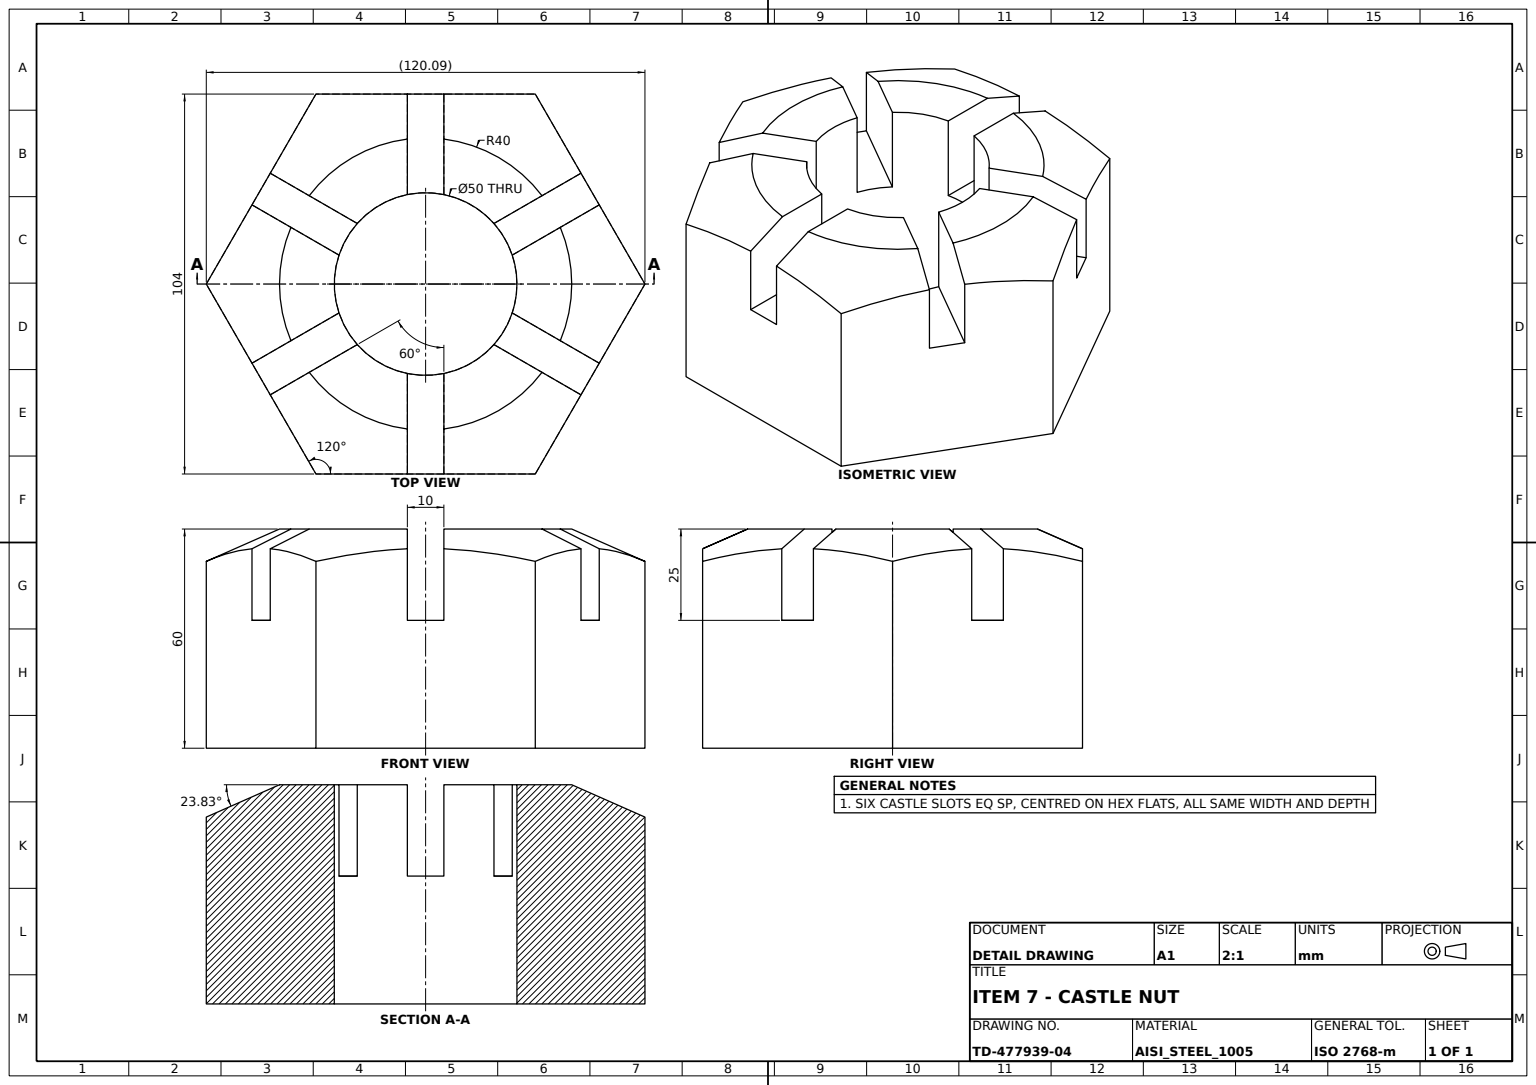
ISO-10303-21;
HEADER;
FILE_DESCRIPTION((''),'2;1');
FILE_NAME('','',(''),(''),'','','');
FILE_SCHEMA(('AUTOMOTIVE_DESIGN'));
ENDSEC;
DATA;
#1=APPLICATION_CONTEXT('');
#2=PRODUCT_CONTEXT('',#1,'mechanical');
#3=PRODUCT('','','',(#2));
#4=PRODUCT_DEFINITION_FORMATION('','',#3);
#5=PRODUCT_DEFINITION_CONTEXT('',#1,'design');
#6=PRODUCT_DEFINITION('','',#4,#5);
#7=PRODUCT_DEFINITION_SHAPE('','',#6);
#8=(LENGTH_UNIT()NAMED_UNIT(*)SI_UNIT(.MILLI.,.METRE.));
#9=(NAMED_UNIT(*)PLANE_ANGLE_UNIT()SI_UNIT($,.RADIAN.));
#10=(NAMED_UNIT(*)SI_UNIT($,.STERADIAN.)SOLID_ANGLE_UNIT());
#11=UNCERTAINTY_MEASURE_WITH_UNIT(LENGTH_MEASURE(0.005),#8,'distance_accuracy_value','');
#12=(GEOMETRIC_REPRESENTATION_CONTEXT(3)GLOBAL_UNCERTAINTY_ASSIGNED_CONTEXT((#11))GLOBAL_UNIT_ASSIGNED_CONTEXT((#8,#9,#10))REPRESENTATION_CONTEXT('',''));
#13=CARTESIAN_POINT('',(-47.533321,21.669873,54.594675));
#14=VERTEX_POINT('',#13);
#15=CARTESIAN_POINT('',(-36.869318,15.513008,60.));
#16=VERTEX_POINT('',#15);
#17=CARTESIAN_POINT('',(-47.533323,21.669874,54.594679));
#18=CARTESIAN_POINT('',(-43.979469,19.618056,56.398596));
#19=CARTESIAN_POINT('',(-40.425051,17.565911,58.201027));
#20=B_SPLINE_CURVE_WITH_KNOTS('',3,(#17,#18,#19,#15),.UNSPECIFIED.,.F.,.F.,(4,4),(0.00000025,0.013448131),.UNSPECIFIED.);
#21=EDGE_CURVE('',#14,#16,#20,.T.);
#22=ORIENTED_EDGE('',*,*,#21,.F.);
#23=CARTESIAN_POINT('',(-60.044428,0.,51.148036));
#24=VERTEX_POINT('',#23);
#25=CARTESIAN_POINT('',(-55.892067,7.1921,52.98179));
#26=CARTESIAN_POINT('',(-51.724583,14.410395,54.240365));
#27=CARTESIAN_POINT('',(-47.533321,21.669873,54.59468));
#28=B_SPLINE_CURVE_WITH_KNOTS('',3,(#23,#25,#26,#27),.UNSPECIFIED.,.F.,.F.,(4,4),(0.000000233,0.025168923),.UNSPECIFIED.);
#29=EDGE_CURVE('',#24,#14,#28,.T.);
#30=ORIENTED_EDGE('',*,*,#29,.F.);
#31=CARTESIAN_POINT('',(-47.533321,-21.669873,54.594675));
#32=VERTEX_POINT('',#31);
#33=CARTESIAN_POINT('',(-47.533321,-21.669873,54.59468));
#34=CARTESIAN_POINT('',(-49.619911,-18.055793,54.418287));
#35=CARTESIAN_POINT('',(-53.818812,-10.783084,53.616325));
#36=CARTESIAN_POINT('',(-57.97964,-3.576317,52.059882));
#37=B_SPLINE_CURVE_WITH_KNOTS('',3,(#33,#34,#35,#36,#23),.UNSPECIFIED.,.F.,.F.,(4,1,4),(0.035155124,0.047629599,0.060104073),.UNSPECIFIED.);
#38=EDGE_CURVE('',#32,#24,#37,.T.);
#39=ORIENTED_EDGE('',*,*,#38,.F.);
#40=CARTESIAN_POINT('',(-36.869318,-15.513008,60.));
#41=VERTEX_POINT('',#40);
#42=CARTESIAN_POINT('',(-40.425051,-17.565911,58.201027));
#43=CARTESIAN_POINT('',(-43.979469,-19.618056,56.398596));
#44=CARTESIAN_POINT('',(-47.533323,-21.669874,54.594679));
#45=B_SPLINE_CURVE_WITH_KNOTS('',3,(#40,#42,#43,#44),.UNSPECIFIED.,.F.,.F.,(4,4),(0.000000498,0.013448379),.UNSPECIFIED.);
#46=EDGE_CURVE('',#41,#32,#45,.T.);
#47=ORIENTED_EDGE('',*,*,#46,.F.);
#48=CARTESIAN_POINT('',(0.,0.,60.));
#49=DIRECTION('',(0.,0.,-1.));
#50=DIRECTION('',(-1.,0.,0.));
#51=AXIS2_PLACEMENT_3D('',#48,#49,#50);
#52=CIRCLE('',#51,40.);
#53=EDGE_CURVE('',#41,#16,#52,.T.);
#54=ORIENTED_EDGE('',*,*,#53,.T.);
#55=EDGE_LOOP('',(#22,#30,#39,#47,#54));
#56=FACE_BOUND('',#55,.T.);
#57=CONICAL_SURFACE('',#51,40.,1.154935364);
#58=ADVANCED_FACE('',(#56),#57,.T.);
#59=CARTESIAN_POINT('',(-5.,-52.,54.59468));
#60=VERTEX_POINT('',#59);
#61=CARTESIAN_POINT('',(-5.,-39.68627,60.));
#62=VERTEX_POINT('',#61);
#63=CARTESIAN_POINT('',(-5.,-47.89636,56.398598));
#64=CARTESIAN_POINT('',(-5.,-43.792065,58.201031));
#65=B_SPLINE_CURVE_WITH_KNOTS('',3,(#59,#63,#64,#61),.UNSPECIFIED.,.F.,.F.,(4,4),(0.047300032,0.060747922),.UNSPECIFIED.);
#66=EDGE_CURVE('',#60,#62,#65,.T.);
#67=ORIENTED_EDGE('',*,*,#66,.T.);
#68=CARTESIAN_POINT('',(-31.869318,-24.173262,60.));
#69=VERTEX_POINT('',#68);
#70=EDGE_CURVE('',#62,#69,#52,.T.);
#71=ORIENTED_EDGE('',*,*,#70,.T.);
#72=CARTESIAN_POINT('',(-42.533321,-30.330127,54.594675));
#73=VERTEX_POINT('',#72);
#74=CARTESIAN_POINT('',(-42.533323,-30.330128,54.594679));
#75=CARTESIAN_POINT('',(-38.979469,-28.27831,56.398596));
#76=CARTESIAN_POINT('',(-35.425051,-26.226165,58.201027));
#77=B_SPLINE_CURVE_WITH_KNOTS('',3,(#74,#75,#76,#68),.UNSPECIFIED.,.F.,.F.,(4,4),(0.00000025,0.013448131),.UNSPECIFIED.);
#78=EDGE_CURVE('',#73,#69,#77,.T.);
#79=ORIENTED_EDGE('',*,*,#78,.F.);
#80=CARTESIAN_POINT('',(-30.022214,-52.,51.148036));
#81=VERTEX_POINT('',#80);
#82=CARTESIAN_POINT('',(-34.174575,-44.8079,52.98179));
#83=CARTESIAN_POINT('',(-38.342059,-37.589605,54.240365));
#84=CARTESIAN_POINT('',(-42.533321,-30.330127,54.59468));
#85=B_SPLINE_CURVE_WITH_KNOTS('',3,(#80,#82,#83,#84),.UNSPECIFIED.,.F.,.F.,(4,4),(0.000000233,0.025168923),.UNSPECIFIED.);
#86=EDGE_CURVE('',#81,#73,#85,.T.);
#87=ORIENTED_EDGE('',*,*,#86,.F.);
#88=CARTESIAN_POINT('',(-25.899769,-52.,52.058307));
#89=CARTESIAN_POINT('',(-17.542965,-52.,53.620138));
#90=CARTESIAN_POINT('',(-9.18181,-52.,54.417922));
#91=B_SPLINE_CURVE_WITH_KNOTS('',3,(#80,#88,#89,#90,#59),.UNSPECIFIED.,.F.,.F.,(4,1,4),(0.051261487,0.063895866,0.076530245),.UNSPECIFIED.);
#92=EDGE_CURVE('',#60,#81,#91,.F.);
#93=ORIENTED_EDGE('',*,*,#92,.F.);
#94=EDGE_LOOP('',(#67,#71,#79,#87,#93));
#95=FACE_BOUND('',#94,.T.);
#96=ADVANCED_FACE('',(#95),#57,.T.);
#97=CARTESIAN_POINT('',(-42.533321,30.330127,54.594675));
#98=VERTEX_POINT('',#97);
#99=CARTESIAN_POINT('',(-30.022214,52.,51.148036));
#100=VERTEX_POINT('',#99);
#101=CARTESIAN_POINT('',(-42.533321,30.330127,54.59468));
#102=CARTESIAN_POINT('',(-40.446731,33.944207,54.418287));
#103=CARTESIAN_POINT('',(-36.24783,41.216916,53.616325));
#104=CARTESIAN_POINT('',(-32.087002,48.423683,52.059882));
#105=B_SPLINE_CURVE_WITH_KNOTS('',3,(#101,#102,#103,#104,#99),.UNSPECIFIED.,.F.,.F.,(4,1,4),(0.035155124,0.047629599,0.060104073),.UNSPECIFIED.);
#106=EDGE_CURVE('',#98,#100,#105,.T.);
#107=ORIENTED_EDGE('',*,*,#106,.F.);
#108=CARTESIAN_POINT('',(-31.869318,24.173262,60.));
#109=VERTEX_POINT('',#108);
#110=CARTESIAN_POINT('',(-35.425051,26.226165,58.201027));
#111=CARTESIAN_POINT('',(-38.979469,28.27831,56.398596));
#112=CARTESIAN_POINT('',(-42.533323,30.330128,54.594679));
#113=B_SPLINE_CURVE_WITH_KNOTS('',3,(#108,#110,#111,#112),.UNSPECIFIED.,.F.,.F.,(4,4),(0.000000498,0.013448379),.UNSPECIFIED.);
#114=EDGE_CURVE('',#109,#98,#113,.T.);
#115=ORIENTED_EDGE('',*,*,#114,.F.);
#116=CARTESIAN_POINT('',(-5.,39.68627,60.));
#117=VERTEX_POINT('',#116);
#118=EDGE_CURVE('',#109,#117,#52,.T.);
#119=ORIENTED_EDGE('',*,*,#118,.T.);
#120=CARTESIAN_POINT('',(-5.,52.,54.59468));
#121=VERTEX_POINT('',#120);
#122=CARTESIAN_POINT('',(-5.,43.792075,58.201027));
#123=CARTESIAN_POINT('',(-5.,47.896365,56.398596));
#124=B_SPLINE_CURVE_WITH_KNOTS('',3,(#116,#122,#123,#120),.UNSPECIFIED.,.F.,.F.,(4,4),(0.029122538,0.04257018),.UNSPECIFIED.);
#125=EDGE_CURVE('',#117,#121,#124,.T.);
#126=ORIENTED_EDGE('',*,*,#125,.T.);
#127=CARTESIAN_POINT('',(-25.899769,52.,52.058307));
#128=CARTESIAN_POINT('',(-17.542965,52.,53.620138));
#129=CARTESIAN_POINT('',(-9.18181,52.,54.417922));
#130=B_SPLINE_CURVE_WITH_KNOTS('',3,(#99,#127,#128,#129,#120),.UNSPECIFIED.,.F.,.F.,(4,1,4),(0.051261487,0.063895866,0.076530245),.UNSPECIFIED.);
#131=EDGE_CURVE('',#100,#121,#130,.T.);
#132=ORIENTED_EDGE('',*,*,#131,.F.);
#133=EDGE_LOOP('',(#107,#115,#119,#126,#132));
#134=FACE_BOUND('',#133,.T.);
#135=ADVANCED_FACE('',(#134),#57,.T.);
#136=CARTESIAN_POINT('',(30.022214,-52.,51.148036));
#137=VERTEX_POINT('',#136);
#138=CARTESIAN_POINT('',(5.,-52.,54.59468));
#139=VERTEX_POINT('',#138);
#140=CARTESIAN_POINT('',(9.183557,-52.,54.417848));
#141=CARTESIAN_POINT('',(17.560472,-52.,53.618083));
#142=CARTESIAN_POINT('',(25.912421,-52.,52.055513));
#143=B_SPLINE_CURVE_WITH_KNOTS('',3,(#138,#140,#141,#142,#136),.UNSPECIFIED.,.F.,.F.,(4,1,4),(0.086598768,0.099232452,0.111866135),.UNSPECIFIED.);
#144=EDGE_CURVE('',#137,#139,#143,.F.);
#145=ORIENTED_EDGE('',*,*,#144,.F.);
#146=CARTESIAN_POINT('',(42.533321,-30.330127,54.594675));
#147=VERTEX_POINT('',#146);
#148=CARTESIAN_POINT('',(42.533321,-30.330127,54.59468));
#149=CARTESIAN_POINT('',(40.446731,-33.944207,54.418287));
#150=CARTESIAN_POINT('',(36.24783,-41.216916,53.616325));
#151=CARTESIAN_POINT('',(32.087002,-48.423683,52.059882));
#152=B_SPLINE_CURVE_WITH_KNOTS('',3,(#148,#149,#150,#151,#136),.UNSPECIFIED.,.F.,.F.,(4,1,4),(0.035155124,0.047629599,0.060104073),.UNSPECIFIED.);
#153=EDGE_CURVE('',#147,#137,#152,.T.);
#154=ORIENTED_EDGE('',*,*,#153,.F.);
#155=CARTESIAN_POINT('',(31.869318,-24.173262,60.));
#156=VERTEX_POINT('',#155);
#157=CARTESIAN_POINT('',(42.533323,-30.330128,54.594679));
#158=CARTESIAN_POINT('',(38.979469,-28.27831,56.398596));
#159=CARTESIAN_POINT('',(35.425051,-26.226165,58.201027));
#160=B_SPLINE_CURVE_WITH_KNOTS('',3,(#157,#158,#159,#155),.UNSPECIFIED.,.F.,.F.,(4,4),(0.00000025,0.013448131),.UNSPECIFIED.);
#161=EDGE_CURVE('',#147,#156,#160,.T.);
#162=ORIENTED_EDGE('',*,*,#161,.T.);
#163=CARTESIAN_POINT('',(5.,-39.68627,60.));
#164=VERTEX_POINT('',#163);
#165=EDGE_CURVE('',#156,#164,#52,.T.);
#166=ORIENTED_EDGE('',*,*,#165,.T.);
#167=CARTESIAN_POINT('',(5.,-43.792073,58.201028));
#168=CARTESIAN_POINT('',(5.,-47.896364,56.398596));
#169=B_SPLINE_CURVE_WITH_KNOTS('',3,(#163,#167,#168,#138),.UNSPECIFIED.,.F.,.F.,(4,4),(0.027022788,0.040470528),.UNSPECIFIED.);
#170=EDGE_CURVE('',#164,#139,#169,.T.);
#171=ORIENTED_EDGE('',*,*,#170,.T.);
#172=EDGE_LOOP('',(#145,#154,#162,#166,#171));
#173=FACE_BOUND('',#172,.T.);
#174=ADVANCED_FACE('',(#173),#57,.T.);
#175=CARTESIAN_POINT('',(60.044428,0.,51.148036));
#176=VERTEX_POINT('',#175);
#177=CARTESIAN_POINT('',(60.044428,0.,0.));
#178=VERTEX_POINT('',#177);
#179=CARTESIAN_POINT('',(60.044428,0.,60.));
#180=VECTOR('',#49,1000.);
#181=LINE('',#179,#180);
#182=EDGE_CURVE('',#176,#178,#181,.T.);
#183=ORIENTED_EDGE('',*,*,#182,.T.);
#184=CARTESIAN_POINT('',(30.022214,52.,0.));
#185=VERTEX_POINT('',#184);
#186=DIRECTION('',(-0.5,0.866025404,0.));
#187=VECTOR('',#186,1000.);
#188=LINE('',#177,#187);
#189=EDGE_CURVE('',#178,#185,#188,.T.);
#190=ORIENTED_EDGE('',*,*,#189,.T.);
#191=CARTESIAN_POINT('',(30.022214,52.,51.148036));
#192=VERTEX_POINT('',#191);
#193=CARTESIAN_POINT('',(30.022214,52.,60.));
#194=LINE('',#193,#180);
#195=EDGE_CURVE('',#192,#185,#194,.T.);
#196=ORIENTED_EDGE('',*,*,#195,.F.);
#197=CARTESIAN_POINT('',(42.533321,30.330127,54.59468));
#198=VERTEX_POINT('',#197);
#199=CARTESIAN_POINT('',(34.174575,44.8079,52.98179));
#200=CARTESIAN_POINT('',(38.342059,37.589605,54.240365));
#201=B_SPLINE_CURVE_WITH_KNOTS('',3,(#191,#199,#200,#197),.UNSPECIFIED.,.F.,.F.,(4,4),(0.000000233,0.025168923),.UNSPECIFIED.);
#202=EDGE_CURVE('',#192,#198,#201,.T.);
#203=ORIENTED_EDGE('',*,*,#202,.T.);
#204=CARTESIAN_POINT('',(42.533321,30.330127,35.));
#205=VERTEX_POINT('',#204);
#206=DIRECTION('',(0.,0.,1.));
#207=VECTOR('',#206,1000.);
#208=LINE('',#204,#207);
#209=EDGE_CURVE('',#205,#198,#208,.T.);
#210=ORIENTED_EDGE('',*,*,#209,.F.);
#211=CARTESIAN_POINT('',(47.533321,21.669873,35.));
#212=VERTEX_POINT('',#211);
#213=LINE('',#211,#187);
#214=EDGE_CURVE('',#212,#205,#213,.T.);
#215=ORIENTED_EDGE('',*,*,#214,.F.);
#216=CARTESIAN_POINT('',(47.533321,21.669873,54.594675));
#217=VERTEX_POINT('',#216);
#218=LINE('',#211,#207);
#219=EDGE_CURVE('',#212,#217,#218,.T.);
#220=ORIENTED_EDGE('',*,*,#219,.T.);
#221=CARTESIAN_POINT('',(47.533321,21.669873,54.59468));
#222=CARTESIAN_POINT('',(49.619911,18.055793,54.418287));
#223=CARTESIAN_POINT('',(53.818812,10.783084,53.616325));
#224=CARTESIAN_POINT('',(57.97964,3.576317,52.059882));
#225=B_SPLINE_CURVE_WITH_KNOTS('',3,(#221,#222,#223,#224,#175),.UNSPECIFIED.,.F.,.F.,(4,1,4),(0.035155124,0.047629599,0.060104073),.UNSPECIFIED.);
#226=EDGE_CURVE('',#217,#176,#225,.T.);
#227=ORIENTED_EDGE('',*,*,#226,.T.);
#228=EDGE_LOOP('',(#183,#190,#196,#203,#210,#215,#220,#227));
#229=FACE_BOUND('',#228,.T.);
#230=DIRECTION('',(-0.866025404,-0.5,0.));
#231=DIRECTION('',(0.5,-0.866025404,0.));
#232=AXIS2_PLACEMENT_3D('',#179,#230,#231);
#233=PLANE('',#232);
#234=ADVANCED_FACE('',(#229),#233,.F.);
#235=CARTESIAN_POINT('',(5.,-24.494897,35.));
#236=VERTEX_POINT('',#235);
#237=CARTESIAN_POINT('',(-5.,-24.494897,35.));
#238=VERTEX_POINT('',#237);
#239=CARTESIAN_POINT('',(0.,0.,35.));
#240=AXIS2_PLACEMENT_3D('',#239,#49,#50);
#241=CIRCLE('',#240,25.);
#242=EDGE_CURVE('',#236,#238,#241,.T.);
#243=ORIENTED_EDGE('',*,*,#242,.T.);
#244=CARTESIAN_POINT('',(-5.,-52.,35.));
#245=VERTEX_POINT('',#244);
#246=CARTESIAN_POINT('',(-5.,-22.912878,35.));
#247=DIRECTION('',(0.,-1.,0.));
#248=VECTOR('',#247,1000.);
#249=LINE('',#246,#248);
#250=EDGE_CURVE('',#245,#238,#249,.F.);
#251=ORIENTED_EDGE('',*,*,#250,.F.);
#252=CARTESIAN_POINT('',(5.,-52.,35.));
#253=VERTEX_POINT('',#252);
#254=DIRECTION('',(1.,0.,0.));
#255=VECTOR('',#254,1000.);
#256=LINE('',#244,#255);
#257=EDGE_CURVE('',#245,#253,#256,.T.);
#258=ORIENTED_EDGE('',*,*,#257,.T.);
#259=DIRECTION('',(0.,1.,0.));
#260=VECTOR('',#259,1000.);
#261=LINE('',#252,#260);
#262=EDGE_CURVE('',#236,#253,#261,.F.);
#263=ORIENTED_EDGE('',*,*,#262,.F.);
#264=EDGE_LOOP('',(#243,#251,#258,#263));
#265=FACE_BOUND('',#264,.T.);
#266=CARTESIAN_POINT('',(0.,1.582019,35.));
#267=AXIS2_PLACEMENT_3D('',#266,#49,#50);
#268=PLANE('',#267);
#269=ADVANCED_FACE('',(#265),#268,.F.);
#270=CARTESIAN_POINT('',(-5.,24.494897,35.));
#271=VERTEX_POINT('',#270);
#272=CARTESIAN_POINT('',(5.,24.494897,35.));
#273=VERTEX_POINT('',#272);
#274=EDGE_CURVE('',#271,#273,#241,.T.);
#275=ORIENTED_EDGE('',*,*,#274,.F.);
#276=CARTESIAN_POINT('',(-5.,24.494897,60.));
#277=VERTEX_POINT('',#276);
#278=CARTESIAN_POINT('',(-5.,24.494897,-20.));
#279=LINE('',#278,#207);
#280=EDGE_CURVE('',#277,#271,#279,.F.);
#281=ORIENTED_EDGE('',*,*,#280,.F.);
#282=CARTESIAN_POINT('',(-18.713203,16.577576,60.));
#283=VERTEX_POINT('',#282);
#284=AXIS2_PLACEMENT_3D('',#48,#49,#254);
#285=CIRCLE('',#284,25.);
#286=EDGE_CURVE('',#283,#277,#285,.T.);
#287=ORIENTED_EDGE('',*,*,#286,.F.);
#288=CARTESIAN_POINT('',(-18.713203,16.577576,35.));
#289=VERTEX_POINT('',#288);
#290=CARTESIAN_POINT('',(-18.713203,16.577576,-20.));
#291=LINE('',#290,#207);
#292=EDGE_CURVE('',#283,#289,#291,.F.);
#293=ORIENTED_EDGE('',*,*,#292,.T.);
#294=CARTESIAN_POINT('',(-23.713203,7.917322,35.));
#295=VERTEX_POINT('',#294);
#296=AXIS2_PLACEMENT_3D('',#239,#206,#254);
#297=CIRCLE('',#296,25.);
#298=EDGE_CURVE('',#289,#295,#297,.T.);
#299=ORIENTED_EDGE('',*,*,#298,.T.);
#300=CARTESIAN_POINT('',(-23.713203,7.917322,60.));
#301=VERTEX_POINT('',#300);
#302=CARTESIAN_POINT('',(-23.713203,7.917322,-20.));
#303=LINE('',#302,#207);
#304=EDGE_CURVE('',#295,#301,#303,.T.);
#305=ORIENTED_EDGE('',*,*,#304,.T.);
#306=CARTESIAN_POINT('',(-23.713203,-7.917322,60.));
#307=VERTEX_POINT('',#306);
#308=EDGE_CURVE('',#307,#301,#285,.T.);
#309=ORIENTED_EDGE('',*,*,#308,.F.);
#310=CARTESIAN_POINT('',(-23.713203,-7.917322,35.));
#311=VERTEX_POINT('',#310);
#312=CARTESIAN_POINT('',(-23.713203,-7.917322,-20.));
#313=LINE('',#312,#207);
#314=EDGE_CURVE('',#307,#311,#313,.F.);
#315=ORIENTED_EDGE('',*,*,#314,.T.);
#316=CARTESIAN_POINT('',(-18.713203,-16.577576,35.));
#317=VERTEX_POINT('',#316);
#318=EDGE_CURVE('',#311,#317,#297,.T.);
#319=ORIENTED_EDGE('',*,*,#318,.T.);
#320=CARTESIAN_POINT('',(-18.713203,-16.577576,60.));
#321=VERTEX_POINT('',#320);
#322=CARTESIAN_POINT('',(-18.713203,-16.577576,-20.));
#323=LINE('',#322,#207);
#324=EDGE_CURVE('',#317,#321,#323,.T.);
#325=ORIENTED_EDGE('',*,*,#324,.T.);
#326=CARTESIAN_POINT('',(-5.,-24.494897,60.));
#327=VERTEX_POINT('',#326);
#328=EDGE_CURVE('',#327,#321,#285,.T.);
#329=ORIENTED_EDGE('',*,*,#328,.F.);
#330=CARTESIAN_POINT('',(-5.,-24.494897,-20.));
#331=LINE('',#330,#207);
#332=EDGE_CURVE('',#238,#327,#331,.T.);
#333=ORIENTED_EDGE('',*,*,#332,.F.);
#334=ORIENTED_EDGE('',*,*,#242,.F.);
#335=CARTESIAN_POINT('',(5.,-24.494897,60.));
#336=VERTEX_POINT('',#335);
#337=CARTESIAN_POINT('',(5.,-24.494897,-20.));
#338=LINE('',#337,#207);
#339=EDGE_CURVE('',#336,#236,#338,.F.);
#340=ORIENTED_EDGE('',*,*,#339,.F.);
#341=CARTESIAN_POINT('',(18.713203,-16.577576,60.));
#342=VERTEX_POINT('',#341);
#343=EDGE_CURVE('',#342,#336,#285,.T.);
#344=ORIENTED_EDGE('',*,*,#343,.F.);
#345=CARTESIAN_POINT('',(18.713203,-16.577576,35.));
#346=VERTEX_POINT('',#345);
#347=CARTESIAN_POINT('',(18.713203,-16.577576,-20.));
#348=LINE('',#347,#207);
#349=EDGE_CURVE('',#346,#342,#348,.T.);
#350=ORIENTED_EDGE('',*,*,#349,.F.);
#351=CARTESIAN_POINT('',(23.713203,-7.917322,35.));
#352=VERTEX_POINT('',#351);
#353=EDGE_CURVE('',#352,#346,#241,.T.);
#354=ORIENTED_EDGE('',*,*,#353,.F.);
#355=CARTESIAN_POINT('',(23.713203,-7.917322,60.));
#356=VERTEX_POINT('',#355);
#357=CARTESIAN_POINT('',(23.713203,-7.917322,-20.));
#358=LINE('',#357,#207);
#359=EDGE_CURVE('',#356,#352,#358,.F.);
#360=ORIENTED_EDGE('',*,*,#359,.F.);
#361=CARTESIAN_POINT('',(23.713203,7.917322,60.));
#362=VERTEX_POINT('',#361);
#363=EDGE_CURVE('',#362,#356,#285,.T.);
#364=ORIENTED_EDGE('',*,*,#363,.F.);
#365=CARTESIAN_POINT('',(23.713203,7.917322,35.));
#366=VERTEX_POINT('',#365);
#367=CARTESIAN_POINT('',(23.713203,7.917322,-20.));
#368=LINE('',#367,#207);
#369=EDGE_CURVE('',#366,#362,#368,.T.);
#370=ORIENTED_EDGE('',*,*,#369,.F.);
#371=CARTESIAN_POINT('',(18.713203,16.577576,35.));
#372=VERTEX_POINT('',#371);
#373=EDGE_CURVE('',#372,#366,#241,.T.);
#374=ORIENTED_EDGE('',*,*,#373,.F.);
#375=CARTESIAN_POINT('',(18.713203,16.577576,60.));
#376=VERTEX_POINT('',#375);
#377=CARTESIAN_POINT('',(18.713203,16.577576,-20.));
#378=LINE('',#377,#207);
#379=EDGE_CURVE('',#376,#372,#378,.F.);
#380=ORIENTED_EDGE('',*,*,#379,.F.);
#381=CARTESIAN_POINT('',(5.,24.494897,60.));
#382=VERTEX_POINT('',#381);
#383=EDGE_CURVE('',#382,#376,#285,.T.);
#384=ORIENTED_EDGE('',*,*,#383,.F.);
#385=CARTESIAN_POINT('',(5.,24.494897,-20.));
#386=LINE('',#385,#207);
#387=EDGE_CURVE('',#273,#382,#386,.T.);
#388=ORIENTED_EDGE('',*,*,#387,.F.);
#389=EDGE_LOOP('',(#275,#281,#287,#293,#299,#305,#309,#315,#319,#325,#329,#333,#334,#340,#344,#350,#354,#360,#364,#370,#374,#380,#384,#388));
#390=FACE_BOUND('',#389,.T.);
#391=CARTESIAN_POINT('',(25.,0.,0.));
#392=VERTEX_POINT('',#391);
#393=CARTESIAN_POINT('',(0.,0.,0.));
#394=AXIS2_PLACEMENT_3D('',#393,#206,#254);
#395=CIRCLE('',#394,25.);
#396=EDGE_CURVE('',#392,#392,#395,.F.);
#397=ORIENTED_EDGE('',*,*,#396,.T.);
#398=EDGE_LOOP('',(#397));
#399=FACE_BOUND('',#398,.T.);
#400=CARTESIAN_POINT('',(0.,0.,-20.));
#401=AXIS2_PLACEMENT_3D('',#400,#206,#254);
#402=CYLINDRICAL_SURFACE('',#401,25.);
#403=ADVANCED_FACE('',(#390,#399),#402,.F.);
#404=ORIENTED_EDGE('',*,*,#318,.F.);
#405=CARTESIAN_POINT('',(-47.533321,-21.669873,35.));
#406=VERTEX_POINT('',#405);
#407=DIRECTION('',(0.866025404,0.5,0.));
#408=VECTOR('',#407,1000.);
#409=LINE('',#405,#408);
#410=EDGE_CURVE('',#311,#406,#409,.F.);
#411=ORIENTED_EDGE('',*,*,#410,.T.);
#412=CARTESIAN_POINT('',(-42.533321,-30.330127,35.));
#413=VERTEX_POINT('',#412);
#414=LINE('',#412,#187);
#415=EDGE_CURVE('',#413,#406,#414,.T.);
#416=ORIENTED_EDGE('',*,*,#415,.F.);
#417=CARTESIAN_POINT('',(-17.343135,-15.786566,35.));
#418=VECTOR('',#230,1000.);
#419=LINE('',#417,#418);
#420=EDGE_CURVE('',#413,#317,#419,.F.);
#421=ORIENTED_EDGE('',*,*,#420,.T.);
#422=EDGE_LOOP('',(#404,#411,#416,#421));
#423=FACE_BOUND('',#422,.T.);
#424=CARTESIAN_POINT('',(1.370069,0.791009,35.));
#425=AXIS2_PLACEMENT_3D('',#424,#206,#254);
#426=PLANE('',#425);
#427=ADVANCED_FACE('',(#423),#426,.T.);
#428=CARTESIAN_POINT('',(5.,52.,35.));
#429=VERTEX_POINT('',#428);
#430=CARTESIAN_POINT('',(5.,22.912878,35.));
#431=LINE('',#430,#260);
#432=EDGE_CURVE('',#429,#273,#431,.F.);
#433=ORIENTED_EDGE('',*,*,#432,.F.);
#434=CARTESIAN_POINT('',(-5.,52.,35.));
#435=VERTEX_POINT('',#434);
#436=VECTOR('',#50,1000.);
#437=LINE('',#428,#436);
#438=EDGE_CURVE('',#429,#435,#437,.T.);
#439=ORIENTED_EDGE('',*,*,#438,.T.);
#440=LINE('',#434,#248);
#441=EDGE_CURVE('',#271,#435,#440,.F.);
#442=ORIENTED_EDGE('',*,*,#441,.F.);
#443=ORIENTED_EDGE('',*,*,#274,.T.);
#444=EDGE_LOOP('',(#433,#439,#442,#443));
#445=FACE_BOUND('',#444,.T.);
#446=CARTESIAN_POINT('',(0.,-1.582019,35.));
#447=AXIS2_PLACEMENT_3D('',#446,#49,#50);
#448=PLANE('',#447);
#449=ADVANCED_FACE('',(#445),#448,.F.);
#450=CARTESIAN_POINT('',(-17.343135,-15.786566,60.));
#451=LINE('',#450,#418);
#452=EDGE_CURVE('',#321,#69,#451,.T.);
#453=ORIENTED_EDGE('',*,*,#452,.T.);
#454=ORIENTED_EDGE('',*,*,#70,.F.);
#455=CARTESIAN_POINT('',(-5.,-22.912878,60.));
#456=LINE('',#455,#248);
#457=EDGE_CURVE('',#327,#62,#456,.T.);
#458=ORIENTED_EDGE('',*,*,#457,.F.);
#459=ORIENTED_EDGE('',*,*,#328,.T.);
#460=EDGE_LOOP('',(#453,#454,#458,#459));
#461=FACE_BOUND('',#460,.T.);
#462=AXIS2_PLACEMENT_3D('',#48,#206,#254);
#463=PLANE('',#462);
#464=ADVANCED_FACE('',(#461),#463,.T.);
#465=ORIENTED_EDGE('',*,*,#457,.T.);
#466=ORIENTED_EDGE('',*,*,#66,.F.);
#467=LINE('',#244,#207);
#468=EDGE_CURVE('',#245,#60,#467,.T.);
#469=ORIENTED_EDGE('',*,*,#468,.F.);
#470=ORIENTED_EDGE('',*,*,#250,.T.);
#471=ORIENTED_EDGE('',*,*,#332,.T.);
#472=EDGE_LOOP('',(#465,#466,#469,#470,#471));
#473=FACE_BOUND('',#472,.T.);
#474=AXIS2_PLACEMENT_3D('',#246,#50,#247);
#475=PLANE('',#474);
#476=ADVANCED_FACE('',(#473),#475,.F.);
#477=ORIENTED_EDGE('',*,*,#298,.F.);
#478=CARTESIAN_POINT('',(-42.533321,30.330127,35.));
#479=VERTEX_POINT('',#478);
#480=DIRECTION('',(0.866025404,-0.5,0.));
#481=VECTOR('',#480,1000.);
#482=LINE('',#478,#481);
#483=EDGE_CURVE('',#289,#479,#482,.F.);
#484=ORIENTED_EDGE('',*,*,#483,.T.);
#485=CARTESIAN_POINT('',(-47.533321,21.669873,35.));
#486=VERTEX_POINT('',#485);
#487=DIRECTION('',(0.5,0.866025404,0.));
#488=VECTOR('',#487,1000.);
#489=LINE('',#485,#488);
#490=EDGE_CURVE('',#486,#479,#489,.T.);
#491=ORIENTED_EDGE('',*,*,#490,.F.);
#492=CARTESIAN_POINT('',(-22.343135,7.126312,35.));
#493=DIRECTION('',(-0.866025404,0.5,0.));
#494=VECTOR('',#493,1000.);
#495=LINE('',#492,#494);
#496=EDGE_CURVE('',#486,#295,#495,.F.);
#497=ORIENTED_EDGE('',*,*,#496,.T.);
#498=EDGE_LOOP('',(#477,#484,#491,#497));
#499=FACE_BOUND('',#498,.T.);
#500=CARTESIAN_POINT('',(1.370069,-0.791009,35.));
#501=AXIS2_PLACEMENT_3D('',#500,#206,#254);
#502=PLANE('',#501);
#503=ADVANCED_FACE('',(#499),#502,.T.);
#504=ORIENTED_EDGE('',*,*,#363,.T.);
#505=CARTESIAN_POINT('',(36.869318,-15.513008,60.));
#506=VERTEX_POINT('',#505);
#507=CARTESIAN_POINT('',(47.533321,-21.669873,60.));
#508=LINE('',#507,#494);
#509=EDGE_CURVE('',#506,#356,#508,.T.);
#510=ORIENTED_EDGE('',*,*,#509,.F.);
#511=CARTESIAN_POINT('',(36.869318,15.513008,60.));
#512=VERTEX_POINT('',#511);
#513=EDGE_CURVE('',#512,#506,#52,.T.);
#514=ORIENTED_EDGE('',*,*,#513,.F.);
#515=CARTESIAN_POINT('',(22.343135,7.126312,60.));
#516=LINE('',#515,#408);
#517=EDGE_CURVE('',#362,#512,#516,.T.);
#518=ORIENTED_EDGE('',*,*,#517,.F.);
#519=EDGE_LOOP('',(#504,#510,#514,#518));
#520=FACE_BOUND('',#519,.T.);
#521=ADVANCED_FACE('',(#520),#463,.T.);
#522=CARTESIAN_POINT('',(42.533321,-30.330127,35.));
#523=VERTEX_POINT('',#522);
#524=LINE('',#522,#207);
#525=EDGE_CURVE('',#523,#147,#524,.T.);
#526=ORIENTED_EDGE('',*,*,#525,.T.);
#527=ORIENTED_EDGE('',*,*,#153,.T.);
#528=CARTESIAN_POINT('',(30.022214,-52.,0.));
#529=VERTEX_POINT('',#528);
#530=CARTESIAN_POINT('',(30.022214,-52.,60.));
#531=LINE('',#530,#180);
#532=EDGE_CURVE('',#137,#529,#531,.T.);
#533=ORIENTED_EDGE('',*,*,#532,.T.);
#534=LINE('',#528,#488);
#535=EDGE_CURVE('',#529,#178,#534,.T.);
#536=ORIENTED_EDGE('',*,*,#535,.T.);
#537=ORIENTED_EDGE('',*,*,#182,.F.);
#538=CARTESIAN_POINT('',(47.533321,-21.669873,54.59468));
#539=VERTEX_POINT('',#538);
#540=CARTESIAN_POINT('',(55.892067,-7.1921,52.98179));
#541=CARTESIAN_POINT('',(51.724583,-14.410395,54.240365));
#542=B_SPLINE_CURVE_WITH_KNOTS('',3,(#175,#540,#541,#538),.UNSPECIFIED.,.F.,.F.,(4,4),(0.000000233,0.025168923),.UNSPECIFIED.);
#543=EDGE_CURVE('',#176,#539,#542,.T.);
#544=ORIENTED_EDGE('',*,*,#543,.T.);
#545=CARTESIAN_POINT('',(47.533321,-21.669873,35.));
#546=VERTEX_POINT('',#545);
#547=LINE('',#545,#207);
#548=EDGE_CURVE('',#546,#539,#547,.T.);
#549=ORIENTED_EDGE('',*,*,#548,.F.);
#550=LINE('',#522,#488);
#551=EDGE_CURVE('',#523,#546,#550,.T.);
#552=ORIENTED_EDGE('',*,*,#551,.F.);
#553=EDGE_LOOP('',(#526,#527,#533,#536,#537,#544,#549,#552));
#554=FACE_BOUND('',#553,.T.);
#555=DIRECTION('',(-0.5,-0.866025404,0.));
#556=AXIS2_PLACEMENT_3D('',#530,#493,#555);
#557=PLANE('',#556);
#558=ADVANCED_FACE('',(#554),#557,.F.);
#559=CARTESIAN_POINT('',(-47.533321,-21.669873,60.));
#560=LINE('',#559,#408);
#561=EDGE_CURVE('',#41,#307,#560,.T.);
#562=ORIENTED_EDGE('',*,*,#561,.F.);
#563=ORIENTED_EDGE('',*,*,#46,.T.);
#564=LINE('',#405,#207);
#565=EDGE_CURVE('',#406,#32,#564,.T.);
#566=ORIENTED_EDGE('',*,*,#565,.F.);
#567=ORIENTED_EDGE('',*,*,#410,.F.);
#568=ORIENTED_EDGE('',*,*,#314,.F.);
#569=EDGE_LOOP('',(#562,#563,#566,#567,#568));
#570=FACE_BOUND('',#569,.T.);
#571=AXIS2_PLACEMENT_3D('',#405,#231,#407);
#572=PLANE('',#571);
#573=ADVANCED_FACE('',(#570),#572,.T.);
#574=CARTESIAN_POINT('',(-5.,52.,60.));
#575=LINE('',#574,#248);
#576=EDGE_CURVE('',#117,#277,#575,.T.);
#577=ORIENTED_EDGE('',*,*,#576,.F.);
#578=ORIENTED_EDGE('',*,*,#118,.F.);
#579=CARTESIAN_POINT('',(-42.533321,30.330127,60.));
#580=LINE('',#579,#481);
#581=EDGE_CURVE('',#109,#283,#580,.T.);
#582=ORIENTED_EDGE('',*,*,#581,.T.);
#583=ORIENTED_EDGE('',*,*,#286,.T.);
#584=EDGE_LOOP('',(#577,#578,#582,#583));
#585=FACE_BOUND('',#584,.T.);
#586=ADVANCED_FACE('',(#585),#463,.T.);
#587=ORIENTED_EDGE('',*,*,#106,.T.);
#588=CARTESIAN_POINT('',(-30.022214,52.,0.));
#589=VERTEX_POINT('',#588);
#590=CARTESIAN_POINT('',(-30.022214,52.,60.));
#591=LINE('',#590,#180);
#592=EDGE_CURVE('',#100,#589,#591,.T.);
#593=ORIENTED_EDGE('',*,*,#592,.T.);
#594=CARTESIAN_POINT('',(-60.044428,0.,0.));
#595=VERTEX_POINT('',#594);
#596=VECTOR('',#555,1000.);
#597=LINE('',#588,#596);
#598=EDGE_CURVE('',#589,#595,#597,.T.);
#599=ORIENTED_EDGE('',*,*,#598,.T.);
#600=CARTESIAN_POINT('',(-60.044428,0.,60.));
#601=LINE('',#600,#180);
#602=EDGE_CURVE('',#24,#595,#601,.T.);
#603=ORIENTED_EDGE('',*,*,#602,.F.);
#604=ORIENTED_EDGE('',*,*,#29,.T.);
#605=LINE('',#485,#207);
#606=EDGE_CURVE('',#486,#14,#605,.T.);
#607=ORIENTED_EDGE('',*,*,#606,.F.);
#608=ORIENTED_EDGE('',*,*,#490,.T.);
#609=LINE('',#478,#207);
#610=EDGE_CURVE('',#479,#98,#609,.T.);
#611=ORIENTED_EDGE('',*,*,#610,.T.);
#612=EDGE_LOOP('',(#587,#593,#599,#603,#604,#607,#608,#611));
#613=FACE_BOUND('',#612,.T.);
#614=AXIS2_PLACEMENT_3D('',#590,#480,#487);
#615=PLANE('',#614);
#616=ADVANCED_FACE('',(#613),#615,.F.);
#617=CARTESIAN_POINT('',(31.869318,24.173262,60.));
#618=VERTEX_POINT('',#617);
#619=CARTESIAN_POINT('',(35.42505,26.226165,58.201027));
#620=CARTESIAN_POINT('',(38.979468,28.278309,56.398596));
#621=B_SPLINE_CURVE_WITH_KNOTS('',3,(#617,#619,#620,#197),.UNSPECIFIED.,.F.,.F.,(4,4),(0.000000498,0.013448377),.UNSPECIFIED.);
#622=EDGE_CURVE('',#618,#198,#621,.T.);
#623=ORIENTED_EDGE('',*,*,#622,.T.);
#624=ORIENTED_EDGE('',*,*,#202,.F.);
#625=CARTESIAN_POINT('',(5.,52.,54.59468));
#626=VERTEX_POINT('',#625);
#627=CARTESIAN_POINT('',(9.183557,52.,54.417848));
#628=CARTESIAN_POINT('',(17.560472,52.,53.618083));
#629=CARTESIAN_POINT('',(25.912421,52.,52.055513));
#630=B_SPLINE_CURVE_WITH_KNOTS('',3,(#625,#627,#628,#629,#191),.UNSPECIFIED.,.F.,.F.,(4,1,4),(0.086598768,0.099232452,0.111866135),.UNSPECIFIED.);
#631=EDGE_CURVE('',#626,#192,#630,.T.);
#632=ORIENTED_EDGE('',*,*,#631,.F.);
#633=CARTESIAN_POINT('',(5.,39.68627,60.));
#634=VERTEX_POINT('',#633);
#635=CARTESIAN_POINT('',(5.,47.896365,56.398596));
#636=CARTESIAN_POINT('',(5.,43.792069,58.20103));
#637=B_SPLINE_CURVE_WITH_KNOTS('',3,(#625,#635,#636,#633),.UNSPECIFIED.,.F.,.F.,(4,4),(0.034307802,0.047755679),.UNSPECIFIED.);
#638=EDGE_CURVE('',#626,#634,#637,.T.);
#639=ORIENTED_EDGE('',*,*,#638,.T.);
#640=EDGE_CURVE('',#634,#618,#52,.T.);
#641=ORIENTED_EDGE('',*,*,#640,.T.);
#642=EDGE_LOOP('',(#623,#624,#632,#639,#641));
#643=FACE_BOUND('',#642,.T.);
#644=ADVANCED_FACE('',(#643),#57,.T.);
#645=LINE('',#434,#207);
#646=EDGE_CURVE('',#435,#121,#645,.T.);
#647=ORIENTED_EDGE('',*,*,#646,.T.);
#648=ORIENTED_EDGE('',*,*,#125,.F.);
#649=ORIENTED_EDGE('',*,*,#576,.T.);
#650=ORIENTED_EDGE('',*,*,#280,.T.);
#651=ORIENTED_EDGE('',*,*,#441,.T.);
#652=EDGE_LOOP('',(#647,#648,#649,#650,#651));
#653=FACE_BOUND('',#652,.T.);
#654=AXIS2_PLACEMENT_3D('',#434,#50,#247);
#655=PLANE('',#654);
#656=ADVANCED_FACE('',(#653),#655,.F.);
#657=ORIENTED_EDGE('',*,*,#209,.T.);
#658=ORIENTED_EDGE('',*,*,#622,.F.);
#659=CARTESIAN_POINT('',(42.533321,30.330127,60.));
#660=LINE('',#659,#418);
#661=EDGE_CURVE('',#618,#376,#660,.T.);
#662=ORIENTED_EDGE('',*,*,#661,.T.);
#663=ORIENTED_EDGE('',*,*,#379,.T.);
#664=LINE('',#204,#418);
#665=EDGE_CURVE('',#372,#205,#664,.F.);
#666=ORIENTED_EDGE('',*,*,#665,.T.);
#667=EDGE_LOOP('',(#657,#658,#662,#663,#666));
#668=FACE_BOUND('',#667,.T.);
#669=AXIS2_PLACEMENT_3D('',#204,#186,#230);
#670=PLANE('',#669);
#671=ADVANCED_FACE('',(#668),#670,.F.);
#672=ORIENTED_EDGE('',*,*,#308,.T.);
#673=CARTESIAN_POINT('',(-22.343135,7.126312,60.));
#674=LINE('',#673,#494);
#675=EDGE_CURVE('',#301,#16,#674,.T.);
#676=ORIENTED_EDGE('',*,*,#675,.T.);
#677=ORIENTED_EDGE('',*,*,#53,.F.);
#678=ORIENTED_EDGE('',*,*,#561,.T.);
#679=EDGE_LOOP('',(#672,#676,#677,#678));
#680=FACE_BOUND('',#679,.T.);
#681=ADVANCED_FACE('',(#680),#463,.T.);
#682=CARTESIAN_POINT('',(47.533323,21.669874,54.594679));
#683=CARTESIAN_POINT('',(43.979469,19.618056,56.398596));
#684=CARTESIAN_POINT('',(40.425051,17.565911,58.201027));
#685=B_SPLINE_CURVE_WITH_KNOTS('',3,(#682,#683,#684,#511),.UNSPECIFIED.,.F.,.F.,(4,4),(0.00000025,0.013448131),.UNSPECIFIED.);
#686=EDGE_CURVE('',#217,#512,#685,.T.);
#687=ORIENTED_EDGE('',*,*,#686,.F.);
#688=ORIENTED_EDGE('',*,*,#219,.F.);
#689=CARTESIAN_POINT('',(22.343135,7.126312,35.));
#690=LINE('',#689,#408);
#691=EDGE_CURVE('',#212,#366,#690,.F.);
#692=ORIENTED_EDGE('',*,*,#691,.T.);
#693=ORIENTED_EDGE('',*,*,#369,.T.);
#694=ORIENTED_EDGE('',*,*,#517,.T.);
#695=EDGE_LOOP('',(#687,#688,#692,#693,#694));
#696=FACE_BOUND('',#695,.T.);
#697=AXIS2_PLACEMENT_3D('',#689,#231,#407);
#698=PLANE('',#697);
#699=ADVANCED_FACE('',(#696),#698,.F.);
#700=CARTESIAN_POINT('',(-30.022214,-52.,0.));
#701=VERTEX_POINT('',#700);
#702=VECTOR('',#231,1000.);
#703=LINE('',#594,#702);
#704=EDGE_CURVE('',#595,#701,#703,.T.);
#705=ORIENTED_EDGE('',*,*,#704,.F.);
#706=ORIENTED_EDGE('',*,*,#598,.F.);
#707=LINE('',#184,#436);
#708=EDGE_CURVE('',#185,#589,#707,.T.);
#709=ORIENTED_EDGE('',*,*,#708,.F.);
#710=ORIENTED_EDGE('',*,*,#189,.F.);
#711=ORIENTED_EDGE('',*,*,#535,.F.);
#712=LINE('',#700,#255);
#713=EDGE_CURVE('',#701,#529,#712,.T.);
#714=ORIENTED_EDGE('',*,*,#713,.F.);
#715=EDGE_LOOP('',(#705,#706,#709,#710,#711,#714));
#716=FACE_BOUND('',#715,.T.);
#717=ORIENTED_EDGE('',*,*,#396,.F.);
#718=EDGE_LOOP('',(#717));
#719=FACE_BOUND('',#718,.T.);
#720=PLANE('',#394);
#721=ADVANCED_FACE('',(#716,#719),#720,.F.);
#722=ORIENTED_EDGE('',*,*,#165,.F.);
#723=CARTESIAN_POINT('',(17.343135,-15.786566,60.));
#724=LINE('',#723,#481);
#725=EDGE_CURVE('',#342,#156,#724,.T.);
#726=ORIENTED_EDGE('',*,*,#725,.F.);
#727=ORIENTED_EDGE('',*,*,#343,.T.);
#728=CARTESIAN_POINT('',(5.,-52.,60.));
#729=LINE('',#728,#260);
#730=EDGE_CURVE('',#164,#336,#729,.T.);
#731=ORIENTED_EDGE('',*,*,#730,.F.);
#732=EDGE_LOOP('',(#722,#726,#727,#731));
#733=FACE_BOUND('',#732,.T.);
#734=ADVANCED_FACE('',(#733),#463,.T.);
#735=ORIENTED_EDGE('',*,*,#114,.T.);
#736=ORIENTED_EDGE('',*,*,#610,.F.);
#737=ORIENTED_EDGE('',*,*,#483,.F.);
#738=ORIENTED_EDGE('',*,*,#292,.F.);
#739=ORIENTED_EDGE('',*,*,#581,.F.);
#740=EDGE_LOOP('',(#735,#736,#737,#738,#739));
#741=FACE_BOUND('',#740,.T.);
#742=AXIS2_PLACEMENT_3D('',#478,#555,#480);
#743=PLANE('',#742);
#744=ADVANCED_FACE('',(#741),#743,.T.);
#745=LINE('',#428,#207);
#746=EDGE_CURVE('',#429,#626,#745,.T.);
#747=ORIENTED_EDGE('',*,*,#746,.T.);
#748=ORIENTED_EDGE('',*,*,#631,.T.);
#749=ORIENTED_EDGE('',*,*,#195,.T.);
#750=ORIENTED_EDGE('',*,*,#708,.T.);
#751=ORIENTED_EDGE('',*,*,#592,.F.);
#752=ORIENTED_EDGE('',*,*,#131,.T.);
#753=ORIENTED_EDGE('',*,*,#646,.F.);
#754=ORIENTED_EDGE('',*,*,#438,.F.);
#755=EDGE_LOOP('',(#747,#748,#749,#750,#751,#752,#753,#754));
#756=FACE_BOUND('',#755,.T.);
#757=AXIS2_PLACEMENT_3D('',#193,#247,#254);
#758=PLANE('',#757);
#759=ADVANCED_FACE('',(#756),#758,.F.);
#760=ORIENTED_EDGE('',*,*,#746,.F.);
#761=ORIENTED_EDGE('',*,*,#432,.T.);
#762=ORIENTED_EDGE('',*,*,#387,.T.);
#763=CARTESIAN_POINT('',(5.,22.912878,60.));
#764=LINE('',#763,#260);
#765=EDGE_CURVE('',#382,#634,#764,.T.);
#766=ORIENTED_EDGE('',*,*,#765,.T.);
#767=ORIENTED_EDGE('',*,*,#638,.F.);
#768=EDGE_LOOP('',(#760,#761,#762,#766,#767));
#769=FACE_BOUND('',#768,.T.);
#770=AXIS2_PLACEMENT_3D('',#430,#254,#259);
#771=PLANE('',#770);
#772=ADVANCED_FACE('',(#769),#771,.F.);
#773=ORIENTED_EDGE('',*,*,#686,.T.);
#774=ORIENTED_EDGE('',*,*,#513,.T.);
#775=CARTESIAN_POINT('',(40.42505,-17.565911,58.201027));
#776=CARTESIAN_POINT('',(43.979468,-19.618055,56.398596));
#777=B_SPLINE_CURVE_WITH_KNOTS('',3,(#505,#775,#776,#538),.UNSPECIFIED.,.F.,.F.,(4,4),(0.000000498,0.013448377),.UNSPECIFIED.);
#778=EDGE_CURVE('',#506,#539,#777,.T.);
#779=ORIENTED_EDGE('',*,*,#778,.T.);
#780=ORIENTED_EDGE('',*,*,#543,.F.);
#781=ORIENTED_EDGE('',*,*,#226,.F.);
#782=EDGE_LOOP('',(#773,#774,#779,#780,#781));
#783=FACE_BOUND('',#782,.T.);
#784=ADVANCED_FACE('',(#783),#57,.T.);
#785=ORIENTED_EDGE('',*,*,#606,.T.);
#786=ORIENTED_EDGE('',*,*,#21,.T.);
#787=ORIENTED_EDGE('',*,*,#675,.F.);
#788=ORIENTED_EDGE('',*,*,#304,.F.);
#789=ORIENTED_EDGE('',*,*,#496,.F.);
#790=EDGE_LOOP('',(#785,#786,#787,#788,#789));
#791=FACE_BOUND('',#790,.T.);
#792=AXIS2_PLACEMENT_3D('',#492,#487,#493);
#793=PLANE('',#792);
#794=ADVANCED_FACE('',(#791),#793,.T.);
#795=ORIENTED_EDGE('',*,*,#324,.F.);
#796=ORIENTED_EDGE('',*,*,#420,.F.);
#797=LINE('',#412,#207);
#798=EDGE_CURVE('',#413,#73,#797,.T.);
#799=ORIENTED_EDGE('',*,*,#798,.T.);
#800=ORIENTED_EDGE('',*,*,#78,.T.);
#801=ORIENTED_EDGE('',*,*,#452,.F.);
#802=EDGE_LOOP('',(#795,#796,#799,#800,#801));
#803=FACE_BOUND('',#802,.T.);
#804=AXIS2_PLACEMENT_3D('',#417,#186,#230);
#805=PLANE('',#804);
#806=ADVANCED_FACE('',(#803),#805,.T.);
#807=ORIENTED_EDGE('',*,*,#373,.T.);
#808=ORIENTED_EDGE('',*,*,#691,.F.);
#809=ORIENTED_EDGE('',*,*,#214,.T.);
#810=ORIENTED_EDGE('',*,*,#665,.F.);
#811=EDGE_LOOP('',(#807,#808,#809,#810));
#812=FACE_BOUND('',#811,.T.);
#813=CARTESIAN_POINT('',(-1.370069,-0.791009,35.));
#814=AXIS2_PLACEMENT_3D('',#813,#49,#50);
#815=PLANE('',#814);
#816=ADVANCED_FACE('',(#812),#815,.F.);
#817=ORIENTED_EDGE('',*,*,#349,.T.);
#818=ORIENTED_EDGE('',*,*,#725,.T.);
#819=ORIENTED_EDGE('',*,*,#161,.F.);
#820=ORIENTED_EDGE('',*,*,#525,.F.);
#821=CARTESIAN_POINT('',(17.343135,-15.786566,35.));
#822=LINE('',#821,#481);
#823=EDGE_CURVE('',#523,#346,#822,.F.);
#824=ORIENTED_EDGE('',*,*,#823,.T.);
#825=EDGE_LOOP('',(#817,#818,#819,#820,#824));
#826=FACE_BOUND('',#825,.T.);
#827=AXIS2_PLACEMENT_3D('',#821,#555,#480);
#828=PLANE('',#827);
#829=ADVANCED_FACE('',(#826),#828,.F.);
#830=ORIENTED_EDGE('',*,*,#765,.F.);
#831=ORIENTED_EDGE('',*,*,#383,.T.);
#832=ORIENTED_EDGE('',*,*,#661,.F.);
#833=ORIENTED_EDGE('',*,*,#640,.F.);
#834=EDGE_LOOP('',(#830,#831,#832,#833));
#835=FACE_BOUND('',#834,.T.);
#836=ADVANCED_FACE('',(#835),#463,.T.);
#837=ORIENTED_EDGE('',*,*,#532,.F.);
#838=ORIENTED_EDGE('',*,*,#144,.T.);
#839=LINE('',#252,#207);
#840=EDGE_CURVE('',#253,#139,#839,.T.);
#841=ORIENTED_EDGE('',*,*,#840,.F.);
#842=ORIENTED_EDGE('',*,*,#257,.F.);
#843=ORIENTED_EDGE('',*,*,#468,.T.);
#844=ORIENTED_EDGE('',*,*,#92,.T.);
#845=CARTESIAN_POINT('',(-30.022214,-52.,60.));
#846=LINE('',#845,#180);
#847=EDGE_CURVE('',#81,#701,#846,.T.);
#848=ORIENTED_EDGE('',*,*,#847,.T.);
#849=ORIENTED_EDGE('',*,*,#713,.T.);
#850=EDGE_LOOP('',(#837,#838,#841,#842,#843,#844,#848,#849));
#851=FACE_BOUND('',#850,.T.);
#852=AXIS2_PLACEMENT_3D('',#845,#259,#50);
#853=PLANE('',#852);
#854=ADVANCED_FACE('',(#851),#853,.F.);
#855=ORIENTED_EDGE('',*,*,#359,.T.);
#856=LINE('',#545,#494);
#857=EDGE_CURVE('',#352,#546,#856,.F.);
#858=ORIENTED_EDGE('',*,*,#857,.T.);
#859=ORIENTED_EDGE('',*,*,#548,.T.);
#860=ORIENTED_EDGE('',*,*,#778,.F.);
#861=ORIENTED_EDGE('',*,*,#509,.T.);
#862=EDGE_LOOP('',(#855,#858,#859,#860,#861));
#863=FACE_BOUND('',#862,.T.);
#864=AXIS2_PLACEMENT_3D('',#545,#487,#493);
#865=PLANE('',#864);
#866=ADVANCED_FACE('',(#863),#865,.F.);
#867=ORIENTED_EDGE('',*,*,#353,.T.);
#868=ORIENTED_EDGE('',*,*,#823,.F.);
#869=ORIENTED_EDGE('',*,*,#551,.T.);
#870=ORIENTED_EDGE('',*,*,#857,.F.);
#871=EDGE_LOOP('',(#867,#868,#869,#870));
#872=FACE_BOUND('',#871,.T.);
#873=CARTESIAN_POINT('',(-1.370069,0.791009,35.));
#874=AXIS2_PLACEMENT_3D('',#873,#49,#50);
#875=PLANE('',#874);
#876=ADVANCED_FACE('',(#872),#875,.F.);
#877=ORIENTED_EDGE('',*,*,#602,.T.);
#878=ORIENTED_EDGE('',*,*,#704,.T.);
#879=ORIENTED_EDGE('',*,*,#847,.F.);
#880=ORIENTED_EDGE('',*,*,#86,.T.);
#881=ORIENTED_EDGE('',*,*,#798,.F.);
#882=ORIENTED_EDGE('',*,*,#415,.T.);
#883=ORIENTED_EDGE('',*,*,#565,.T.);
#884=ORIENTED_EDGE('',*,*,#38,.T.);
#885=EDGE_LOOP('',(#877,#878,#879,#880,#881,#882,#883,#884));
#886=FACE_BOUND('',#885,.T.);
#887=AXIS2_PLACEMENT_3D('',#600,#407,#186);
#888=PLANE('',#887);
#889=ADVANCED_FACE('',(#886),#888,.F.);
#890=ORIENTED_EDGE('',*,*,#262,.T.);
#891=ORIENTED_EDGE('',*,*,#840,.T.);
#892=ORIENTED_EDGE('',*,*,#170,.F.);
#893=ORIENTED_EDGE('',*,*,#730,.T.);
#894=ORIENTED_EDGE('',*,*,#339,.T.);
#895=EDGE_LOOP('',(#890,#891,#892,#893,#894));
#896=FACE_BOUND('',#895,.T.);
#897=AXIS2_PLACEMENT_3D('',#252,#254,#259);
#898=PLANE('',#897);
#899=ADVANCED_FACE('',(#896),#898,.F.);
#900=CLOSED_SHELL('',(#58,#96,#135,#174,#234,#269,#403,#427,#449,#464,#476,#503,#521,#558,#573,#586,#616,#644,#656,#671,#681,#699,#721,#734,#744,#759,#772,#784,#794,#806,#816,#829,#836,#854,#866,#876,#889,#899));
#901=MANIFOLD_SOLID_BREP('',#900);
#902=ADVANCED_BREP_SHAPE_REPRESENTATION('',(#901),#12);
#903=SHAPE_DEFINITION_REPRESENTATION(#7,#902);
ENDSEC;
END-ISO-10303-21;
